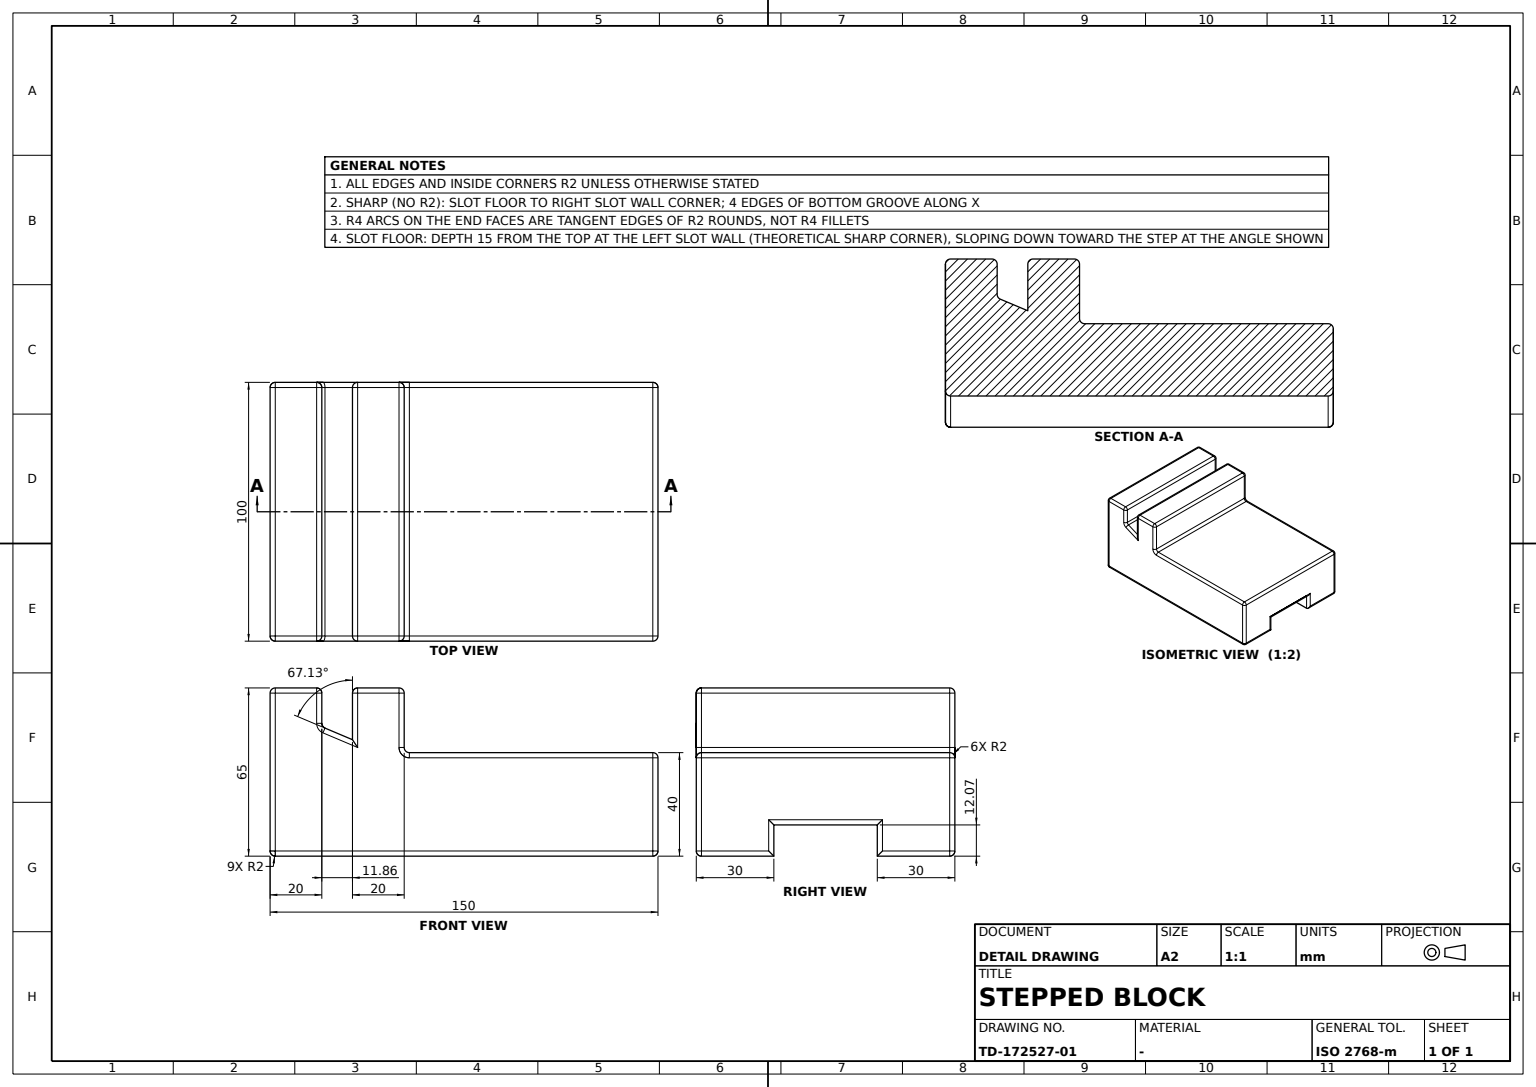
solid
v1 (-73,-2,-32.5)
v2 (-75,-2,-30.5)
e1 v1 v2 CIRCLE(AX(P(-73,-2,-30.5),D(0,-1,0),D(0,0,-1)),2) rev
v3 (-73,0,-30.5)
e2 v3 v2 CIRCLE(AX(P(-73,-2,-30.5),D(0,0,1),D(1,0,0)),2)
e3 v3 v1 CIRCLE(AX(P(-73,-2,-30.5),D(-1,0,0),D(0,0,1)),2)
face SPHERE(AX(P(-73,-2,-30.5),D(-0.707106781,0,0.707106781),D(0,-1,0)),2) [e1 -e2 e3]
v4 (-41.144917,-100,30.5)
v5 (-25.144917,-100,30.5)
e4 v4 v5 LINE
v6 (-25.144917,-98,32.5)
e5 v6 v5 CIRCLE(AX(P(-25.144917,-98,30.5),D(-1,0,0),D(0,0,1)),2) rev
v7 (-41.144917,-98,32.5)
e6 v7 v6 LINE
e7 v7 v4 CIRCLE(AX(P(-41.144917,-98,30.5),D(-1,0,0),D(0,0,1)),2) rev
face CYL(AX(P(1,-98,30.5),D(-1,0,0),D(0,-1,0)),2) [e4 -e5 -e6 e7]
v8 (-23.144917,-98,9.5)
v9 (-21.144917,-98,7.5)
e8 v8 v9 CIRCLE(AX(P(-21.144917,-98,9.5),D(0,-1,0),D(0,0,-1)),2)
v10 (-25.144917,-100,9.5)
e9 v8 v10 CIRCLE(AX(P(-25.144917,-98,9.5),D(0,0,-1),D(-1,0,0)),2)
v11 (-21.144917,-100,5.5)
e10 v10 v11 CIRCLE(AX(P(-21.144917,-100,9.5),D(0,-1,0),D(0,0,-1)),4)
e11 v9 v11 CIRCLE(AX(P(-21.144917,-98,5.5),D(1,0,0),D(0,0,-1)),2)
face TORUS(AX(P(-21.144917,-98,9.5),D(0,-1,0),D(0.051622816,0,0.998666654)),4,2) [-e8 e9 e10 -e11]
v12 (-43.144917,-98,30.5)
e12 v7 v12 CIRCLE(AX(P(-41.144917,-98,30.5),D(0,-1,0),D(0,0,-1)),2)
e13 v12 v4 CIRCLE(AX(P(-41.144917,-98,30.5),D(0,0,1),D(1,0,0)),2)
face SPHERE(AX(P(-41.144917,-98,30.5),D(0,0,1),D(-0.965925826,0.258819045,0)),2) [e12 e13 -e7]
v13 (-23.144917,-98,30.5)
e14 v13 v6 CIRCLE(AX(P(-25.144917,-98,30.5),D(0,-1,0),D(0,0,-1)),2)
e15 v13 v5 CIRCLE(AX(P(-25.144917,-98,30.5),D(0,0,-1),D(-1,0,0)),2)
face SPHERE(AX(P(-25.144917,-98,30.5),D(0,-1,0),D(0.965925826,0,-0.258819045)),2) [e14 e5 -e15]
v14 (-73,0,30.5)
e16 v3 v14 LINE
v15 (-57,0,30.5)
e17 v14 v15 LINE
v16 (-57,0,18.827085)
e18 v15 v16 LINE
v17 (-54.554442,0,15.141477)
e19 v16 v17 CIRCLE(AX(P(-53,0,18.827085),D(0,-1,0),D(0,0,-1)),4)
v18 (-41.144917,0,9.485875)
e20 v17 v18 LINE
v19 (-41.144917,0,30.5)
e21 v18 v19 LINE
v20 (-25.144917,0,30.5)
e22 v19 v20 LINE
v21 (-25.144917,0,9.5)
e23 v20 v21 LINE
v22 (-21.144917,0,5.5)
e24 v21 v22 CIRCLE(AX(P(-21.144917,0,9.5),D(0,-1,0),D(0,0,-1)),4)
v23 (73,0,5.5)
e25 v22 v23 LINE
v24 (73,0,-30.5)
e26 v23 v24 LINE
e27 v24 v3 LINE
face PLANE(AX(P(0,0,0),D(0,1,0),D(-1,0,0))) [e16 e17 e18 e19 e20 e21 e22 e23 e24 e25 e26 e27]
v25 (73,-30,-20.431749)
v26 (-73,-30,-20.431749)
e28 v25 v26 LINE
v27 (-73,-30,-32.5)
e29 v26 v27 LINE
v28 (73,-30,-32.5)
e30 v28 v27 LINE
e31 v25 v28 LINE
face PLANE(AX(P(75,-30,-20.431749),D(0,1,0),D(0,0,-1))) rev [e28 e29 -e30 -e31]
v29 (73,-70,-20.431749)
v30 (-73,-70,-20.431749)
e32 v29 v30 LINE
v31 (73,-70,-32.5)
e33 v31 v29 LINE
v32 (-73,-70,-32.5)
e34 v31 v32 LINE
e35 v32 v30 LINE
face PLANE(AX(P(75,-70,-32.5),D(0,-1,0),D(0,0,1))) rev [-e32 -e33 e34 e35]
v33 (75,-98,-30.5)
v34 (73,-98,-32.5)
e36 v33 v34 CIRCLE(AX(P(73,-98,-30.5),D(0,1,0),D(0,0,1)),2)
e37 v34 v31 LINE
v35 (75,-72,-30.5)
e38 v35 v31 ELLIPSE(AX(P(73,-72,-30.5),D(0,0.707106781,0.707106781),D(0,-0.707106781,0.707106781)),2.828427,2)
e39 v33 v35 LINE
face CYL(AX(P(73,-50,-30.5),D(0,1,0),D(1,0,0)),2) [e36 e37 -e38 -e39]
v36 (-75,-98,-30.5)
v37 (-75,-98,30.5)
e40 v36 v37 LINE
v38 (-75,-2,30.5)
e41 v37 v38 LINE
e42 v2 v38 LINE
v39 (-75,-28,-30.5)
e43 v2 v39 LINE
v40 (-75,-28,-18.431749)
e44 v40 v39 LINE
v41 (-75,-72,-18.431749)
e45 v41 v40 LINE
v42 (-75,-72,-30.5)
e46 v42 v41 LINE
e47 v42 v36 LINE
face PLANE(AX(P(-75,0,-32.5),D(1,0,0),D(0,0,1))) rev [e40 e41 -e42 e43 -e44 -e45 -e46 e47]
v43 (75,-2,5.5)
v44 (73,-2,7.5)
e48 v43 v44 CIRCLE(AX(P(73,-2,5.5),D(0,-1,0),D(0,0,-1)),2)
e49 v43 v23 CIRCLE(AX(P(73,-2,5.5),D(0,0,-1),D(-1,0,0)),2) rev
e50 v44 v23 CIRCLE(AX(P(73,-2,5.5),D(1,0,0),D(0,0,-1)),2) rev
face SPHERE(AX(P(73,-2,5.5),D(0,1,0),D(0.965925826,0,-0.258819045)),2) [-e48 e49 -e50]
v45 (-53.777221,-2,16.984281)
v46 (-53.777221,-98,16.984281)
e51 v45 v46 LINE
v47 (-43.144917,-98,12.5)
e52 v47 v46 LINE
v48 (-43.144917,-2,12.5)
e53 v48 v47 LINE
e54 v45 v48 LINE
face PLANE(AX(P(-55,0,17.5),D(-0.388610552,0,-0.921402105),D(0.921402105,0,-0.388610552))) rev [e51 -e52 -e53 -e54]
v49 (-41.144917,-100,9.485875)
e55 v49 v4 LINE
e56 v47 v12 LINE
e57 v47 v49 ELLIPSE(AX(P(-41.144917,-98,9.485875),D(-0.833249828,0,-0.552896667),D(-0.552896667,0,0.833249828)),3.617312,2) rev
face CYL(AX(P(-41.144917,-98,0),D(0,0,1),D(0,-1,0)),2) [e55 -e13 -e56 e57]
v50 (75,-98,5.5)
v51 (73,-100,5.5)
e58 v50 v51 CIRCLE(AX(P(73,-98,5.5),D(0,0,-1),D(-1,0,0)),2)
v52 (73,-100,-30.5)
e59 v51 v52 LINE
e60 v33 v52 CIRCLE(AX(P(73,-98,-30.5),D(0,0,-1),D(-1,0,0)),2)
e61 v50 v33 LINE
face CYL(AX(P(73,-98,1),D(0,0,-1),D(1,0,0)),2) [e58 e59 -e60 -e61]
v53 (-55,-2,18.827085)
e62 v53 v45 CIRCLE(AX(P(-53,-2,18.827085),D(0,-1,0),D(0,0,-1)),2)
e63 v45 v17 CIRCLE(AX(P(-54.554442,-2,15.141477),D(0.921402105,0,-0.388610552),D(-0.388610552,0,-0.921402105)),2) rev
e64 v53 v16 CIRCLE(AX(P(-57,-2,18.827085),D(0,0,-1),D(-1,0,0)),2) rev
face TORUS(AX(P(-53,-2,18.827085),D(0,-1,0),D(-0.231621746,0,0.972805925)),4,2) [e62 e63 -e19 -e64]
e65 v1 v27 LINE
e66 v39 v27 ELLIPSE(AX(P(-73,-28,-30.5),D(0,0.707106781,-0.707106781),D(0,-0.707106781,-0.707106781)),2.828427,2) rev
face CYL(AX(P(-73,-50,-30.5),D(0,-1,0),D(0,0,-1)),2) [-e43 -e1 e65 -e66]
v54 (-43.144917,-2,30.5)
e67 v48 v54 LINE
e68 v19 v54 CIRCLE(AX(P(-41.144917,-2,30.5),D(0,0,1),D(1,0,0)),2)
e69 v18 v48 ELLIPSE(AX(P(-41.144917,-2,9.485875),D(0.833249828,0,0.552896667),D(-0.552896667,0,0.833249828)),3.617312,2)
face CYL(AX(P(-41.144917,-2,1),D(0,0,1),D(-1,0,0)),2) [e67 -e68 -e21 e69]
v55 (-25.144917,-2,32.5)
e70 v55 v6 LINE
v56 (-23.144917,-2,30.5)
e71 v56 v13 LINE
e72 v56 v55 CIRCLE(AX(P(-25.144917,-2,30.5),D(0,-1,0),D(0,0,-1)),2)
face CYL(AX(P(-25.144917,-50,30.5),D(0,-1,0),D(0,0,1)),2) [e70 -e14 -e71 e72]
v57 (-73,-100,-30.5)
e73 v36 v57 CIRCLE(AX(P(-73,-98,-30.5),D(0,0,1),D(1,0,0)),2)
v58 (-73,-100,30.5)
e74 v57 v58 LINE
e75 v37 v58 CIRCLE(AX(P(-73,-98,30.5),D(0,0,1),D(1,0,0)),2)
face CYL(AX(P(-73,-98,0),D(0,0,1),D(0,-1,0)),2) [-e40 e73 e74 -e75]
v59 (73,-98,7.5)
e76 v50 v59 CIRCLE(AX(P(73,-98,5.5),D(0,-1,0),D(0,0,-1)),2)
e77 v59 v51 CIRCLE(AX(P(73,-98,5.5),D(1,0,0),D(0,0,-1)),2)
face SPHERE(AX(P(73,-98,5.5),D(0,-1,0),D(0.965925826,0,-0.258819045)),2) [-e58 e76 e77]
e78 v40 v26 ELLIPSE(AX(P(-73,-28,-18.431749),D(0,0.707106781,-0.707106781),D(0,0.707106781,0.707106781)),2.828427,2) rev
face CYL(AX(P(-73,-28,-1),D(0,0,-1),D(0,-1,0)),2) [-e29 -e78 e44 e66]
v60 (-73,-98,-32.5)
e79 v60 v36 CIRCLE(AX(P(-73,-98,-30.5),D(0,-1,0),D(0,0,-1)),2) rev
e80 v60 v57 CIRCLE(AX(P(-73,-98,-30.5),D(-1,0,0),D(0,0,1)),2)
face SPHERE(AX(P(-73,-98,-30.5),D(-0.707106781,0,0.707106781),D(0,-1,0)),2) [-e79 e80 -e73]
v61 (-73,-98,32.5)
v62 (-73,-2,32.5)
e81 v61 v62 LINE
e82 v38 v62 CIRCLE(AX(P(-73,-2,30.5),D(0,1,0),D(0,0,1)),2)
e83 v37 v61 CIRCLE(AX(P(-73,-98,30.5),D(0,1,0),D(0,0,1)),2)
face CYL(AX(P(-73,-51,30.5),D(0,1,0),D(-1,0,0)),2) [e81 -e82 -e41 e83]
v63 (-41.144917,-2,32.5)
e84 v63 v7 LINE
e85 v63 v54 CIRCLE(AX(P(-41.144917,-2,30.5),D(0,-1,0),D(0,0,-1)),2)
e86 v54 v12 LINE
face CYL(AX(P(-41.144917,-46.916496,30.5),D(0,-1,0),D(0,0,1)),2) [-e84 e85 e86 -e12]
e87 v52 v57 LINE
e88 v34 v60 LINE
e89 v34 v52 CIRCLE(AX(P(73,-98,-30.5),D(-1,0,0),D(0,0,1)),2)
face CYL(AX(P(0,-98,-30.5),D(-1,0,0),D(0,-1,0)),2) [e87 -e80 -e88 e89]
e90 v42 v32 ELLIPSE(AX(P(-73,-72,-30.5),D(0,-0.707106781,-0.707106781),D(0,-0.707106781,0.707106781)),2.828427,2)
e91 v32 v60 LINE
face CYL(AX(P(-73,-50,-30.5),D(0,-1,0),D(0,0,-1)),2) [e79 -e47 e90 e91]
v64 (-55,-2,30.5)
v65 (-55,-98,30.5)
e92 v64 v65 LINE
v66 (-57,-2,32.5)
e93 v64 v66 CIRCLE(AX(P(-57,-2,30.5),D(0,-1,0),D(0,0,-1)),2)
v67 (-57,-98,32.5)
e94 v66 v67 LINE
e95 v65 v67 CIRCLE(AX(P(-57,-98,30.5),D(0,-1,0),D(0,0,-1)),2)
face CYL(AX(P(-57,-46.912746,30.5),D(0,-1,0),D(1,0,0)),2) [-e92 e93 e94 -e95]
e96 v56 v20 CIRCLE(AX(P(-25.144917,-2,30.5),D(0,0,-1),D(-1,0,0)),2) rev
e97 v55 v20 CIRCLE(AX(P(-25.144917,-2,30.5),D(1,0,0),D(0,0,-1)),2) rev
face SPHERE(AX(P(-25.144917,-2,30.5),D(0,1,0),D(0.965925826,0,-0.258819045)),2) [-e72 e96 -e97]
v68 (-23.144917,-2,9.5)
e98 v56 v68 LINE
e99 v68 v21 CIRCLE(AX(P(-25.144917,-2,9.5),D(0,0,-1),D(-1,0,0)),2) rev
face CYL(AX(P(-25.144917,-2,1),D(0,0,-1),D(1,0,0)),2) [e98 e99 -e23 -e96]
v69 (75,-28,-30.5)
v70 (75,-2,-30.5)
e100 v69 v70 LINE
e101 v43 v70 LINE
e102 v43 v50 LINE
v71 (75,-72,-18.431749)
e103 v35 v71 LINE
v72 (75,-28,-18.431749)
e104 v71 v72 LINE
e105 v72 v69 LINE
face PLANE(AX(P(75,0,7.5),D(-1,0,0),D(0,0,-1))) rev [e100 -e101 e102 e61 e39 e103 e104 e105]
v73 (73,-2,-32.5)
e106 v24 v73 CIRCLE(AX(P(73,-2,-30.5),D(-1,0,0),D(0,0,1)),2)
e107 v73 v1 LINE
face CYL(AX(P(0,-2,-30.5),D(-1,0,0),D(0,0,-1)),2) [-e27 e106 e107 -e3]
e108 v15 v66 CIRCLE(AX(P(-57,-2,30.5),D(1,0,0),D(0,0,-1)),2)
e109 v14 v62 CIRCLE(AX(P(-73,-2,30.5),D(1,0,0),D(0,0,-1)),2)
e110 v62 v66 LINE
face CYL(AX(P(0,-2,30.5),D(1,0,0),D(0,0,1)),2) [-e108 -e17 e109 e110]
e111 v70 v24 CIRCLE(AX(P(73,-2,-30.5),D(0,0,-1),D(-1,0,0)),2) rev
e112 v70 v73 CIRCLE(AX(P(73,-2,-30.5),D(0,1,0),D(0,0,1)),2)
face SPHERE(AX(P(73,-2,-30.5),D(1,0,0),D(0,0.965925826,0.258819045)),2) [-e106 -e111 e112]
v74 (-57,-100,30.5)
e113 v65 v74 CIRCLE(AX(P(-57,-98,30.5),D(0,0,-1),D(-1,0,0)),2)
v75 (-57,-100,18.827085)
e114 v74 v75 LINE
v76 (-55,-98,18.827085)
e115 v75 v76 CIRCLE(AX(P(-57,-98,18.827085),D(0,0,-1),D(-1,0,0)),2) rev
e116 v65 v76 LINE
face CYL(AX(P(-57,-98,0),D(0,0,-1),D(0,-1,0)),2) [e113 e114 e115 -e116]
face SPHERE(AX(P(73,-98,-30.5),D(1,0,0),D(0,0.258819045,-0.965925826)),2) [e60 -e89 -e36]
e117 v41 v30 ELLIPSE(AX(P(-73,-72,-18.431749),D(0,0.707106781,0.707106781),D(0,0.707106781,-0.707106781)),2.828427,2) rev
face CYL(AX(P(-73,-72,-1),D(0,0,1),D(0,1,0)),2) [e117 -e35 -e90 e46]
face PLANE(AX(P(75,0,-32.5),D(0,0,1),D(-1,0,0))) rev [-e37 e88 -e91 -e34]
e118 v68 v8 LINE
e119 v13 v8 LINE
face PLANE(AX(P(-23.144917,0,32.5),D(-1,0,0),D(0,0,-1))) rev [-e118 -e98 e71 e119]
e120 v9 v59 LINE
e121 v44 v59 LINE
v77 (-21.144917,-2,7.5)
e122 v77 v44 LINE
e123 v77 v9 LINE
face PLANE(AX(P(-23.144917,0,7.5),D(0,0,-1),D(1,0,0))) rev [e120 -e121 -e122 e123]
e124 v38 v14 CIRCLE(AX(P(-73,-2,30.5),D(0,0,1),D(1,0,0)),2) rev
face CYL(AX(P(-73,-2,0),D(0,0,1),D(-1,0,0)),2) [e2 e42 e124 -e16]
face CYL(AX(P(73,-50,5.5),D(0,-1,0),D(0,0,1)),2) [-e102 e48 e121 -e76]
face SPHERE(AX(P(-73,-2,30.5),D(-1,0,0),D(0,0.965925826,-0.258819045)),2) [e82 -e109 -e124]
e125 v5 v10 LINE
face CYL(AX(P(-25.144917,-98,1),D(0,0,-1),D(1,0,0)),2) [e15 e125 -e9 -e119]
e126 v63 v55 LINE
e127 v63 v19 CIRCLE(AX(P(-41.144917,-2,30.5),D(1,0,0),D(0,0,-1)),2) rev
face CYL(AX(P(0,-2,30.5),D(1,0,0),D(0,0,1)),2) [e126 e97 -e22 -e127]
e128 v46 v76 CIRCLE(AX(P(-53,-98,18.827085),D(0,-1,0),D(0,0,-1)),2) rev
v78 (-54.554442,-100,15.141477)
e129 v78 v75 CIRCLE(AX(P(-53,-100,18.827085),D(0,1,0),D(0,0,1)),4)
e130 v78 v46 CIRCLE(AX(P(-54.554442,-98,15.141477),D(-0.921402105,0,0.388610552),D(0.388610552,0,0.921402105)),2)
face TORUS(AX(P(-53,-98,18.827085),D(0,1,0),D(0.806334772,0,-0.591459411)),4,2) [e128 -e115 -e129 e130]
face CYL(AX(P(73,-2,1),D(0,0,-1),D(1,0,0)),2) [e111 -e26 -e49 e101]
e131 v67 v61 LINE
face PLANE(AX(P(-75,0,32.5),D(0,0,-1),D(1,0,0))) rev [-e81 -e131 -e94 -e110]
e132 v30 v26 LINE
face CYL(AX(P(-73,-50,-18.431749),D(0,1,0),D(0,0,-1)),2) [-e132 -e117 e45 e78]
e133 v64 v15 CIRCLE(AX(P(-57,-2,30.5),D(0,0,-1),D(-1,0,0)),2) rev
face SPHERE(AX(P(-57,-2,30.5),D(1,0,0),D(0,0.965925826,-0.258819045)),2) [e108 -e93 e133]
e134 v29 v71 ELLIPSE(AX(P(73,-72,-18.431749),D(0,0.707106781,0.707106781),D(0,0.707106781,-0.707106781)),2.828427,2) rev
face CYL(AX(P(73,-72,-13.5),D(0,0,1),D(1,0,0)),2) [e33 e134 -e103 e38]
e135 v29 v25 LINE
e136 v25 v72 ELLIPSE(AX(P(73,-28,-18.431749),D(0,0.707106781,-0.707106781),D(0,-0.707106781,-0.707106781)),2.828427,2) rev
face CYL(AX(P(73,-50,-18.431749),D(0,1,0),D(1,0,0)),2) [-e134 e135 e136 -e104]
e137 v11 v51 LINE
e138 v49 v78 LINE
e139 v74 v58 LINE
face PLANE(AX(P(0,-100,0),D(0,1,0),D(-1,0,0))) rev [-e59 -e137 -e10 -e125 -e4 -e55 e138 e129 -e114 e139 -e74 -e87]
e140 v68 v77 CIRCLE(AX(P(-21.144917,-2,9.5),D(0,-1,0),D(0,0,-1)),2)
face CYL(AX(P(-21.144917,-50,9.5),D(0,-1,0),D(-1,0,0)),2) rev [-e123 -e140 e118 e8]
face SPHERE(AX(P(-41.144917,-2,30.5),D(0,0,1),D(0.258819045,0.965925826,0)),2) [-e85 e127 e68]
face CYL(AX(P(1,-98,5.5),D(1,0,0),D(0,0,1)),2) [e137 -e77 -e120 e11]
e141 v64 v53 LINE
e142 v53 v76 LINE
face PLANE(AX(P(-55,0,32.5),D(-1,0,0),D(0,0,-1))) rev [-e141 e92 e116 -e142]
e143 v28 v73 LINE
e144 v69 v28 ELLIPSE(AX(P(73,-28,-30.5),D(0,0.707106781,-0.707106781),D(0,0.707106781,0.707106781)),2.828427,2)
face CYL(AX(P(73,-50,-30.5),D(0,1,0),D(1,0,0)),2) [e143 -e112 -e100 e144]
face CYL(AX(P(73,-28,-12.5),D(0,0,-1),D(1,0,0)),2) [-e144 -e105 -e136 e31]
face PLANE(AX(P(-75,0,32.5),D(0,0,-1),D(1,0,0))) rev [-e126 e84 e6 -e70]
face PLANE(AX(P(-43.144917,0,12.5),D(1,0,0),D(0,0,1))) rev [-e86 -e67 e53 e56]
e145 v77 v22 CIRCLE(AX(P(-21.144917,-2,5.5),D(1,0,0),D(0,0,-1)),2) rev
face CYL(AX(P(1,-2,5.5),D(1,0,0),D(0,0,1)),2) [-e25 -e145 e122 e50]
e146 v58 v61 CIRCLE(AX(P(-73,-98,30.5),D(-1,0,0),D(0,0,1)),2)
e147 v74 v67 CIRCLE(AX(P(-57,-98,30.5),D(-1,0,0),D(0,0,1)),2)
face CYL(AX(P(1,-98,30.5),D(-1,0,0),D(0,-1,0)),2) [-e146 -e139 e147 e131]
face CYL(AX(P(-10.731465,-2,-3.341302),D(0.921402105,0,-0.388610552),D(0.388610552,0,0.921402105)),2) [-e20 -e63 e54 -e69]
face CYL(AX(P(-57,-2,1),D(0,0,-1),D(1,0,0)),2) [-e133 e141 e64 -e18]
face TORUS(AX(P(-21.144917,-2,9.5),D(0,-1,0),D(-0.383347987,0,0.923603985)),4,2) [-e99 e140 e145 -e24]
face CYL(AX(P(-7.886244,-98,-4.541302),D(-0.921402105,0,0.388610552),D(0,-1,0)),2) [-e57 e52 -e130 -e138]
face SPHERE(AX(P(-73,-98,30.5),D(0,0,1),D(-0.965925826,0.258819045,0)),2) [e146 -e83 e75]
face SPHERE(AX(P(-57,-98,30.5),D(0,0,1),D(0.965925826,0.258819045,0)),2) [-e147 -e113 e95]
face PLANE(AX(P(75,-70,-20.431749),D(0,0,1),D(0,1,0))) rev [-e135 e32 e132 -e28]
face PLANE(AX(P(75,0,-32.5),D(0,0,1),D(-1,0,0))) rev [-e107 -e143 e30 -e65]
face CYL(AX(P(-53,-50,18.827085),D(0,-1,0),D(-1,0,0)),2) rev [e142 -e128 -e51 -e62]
